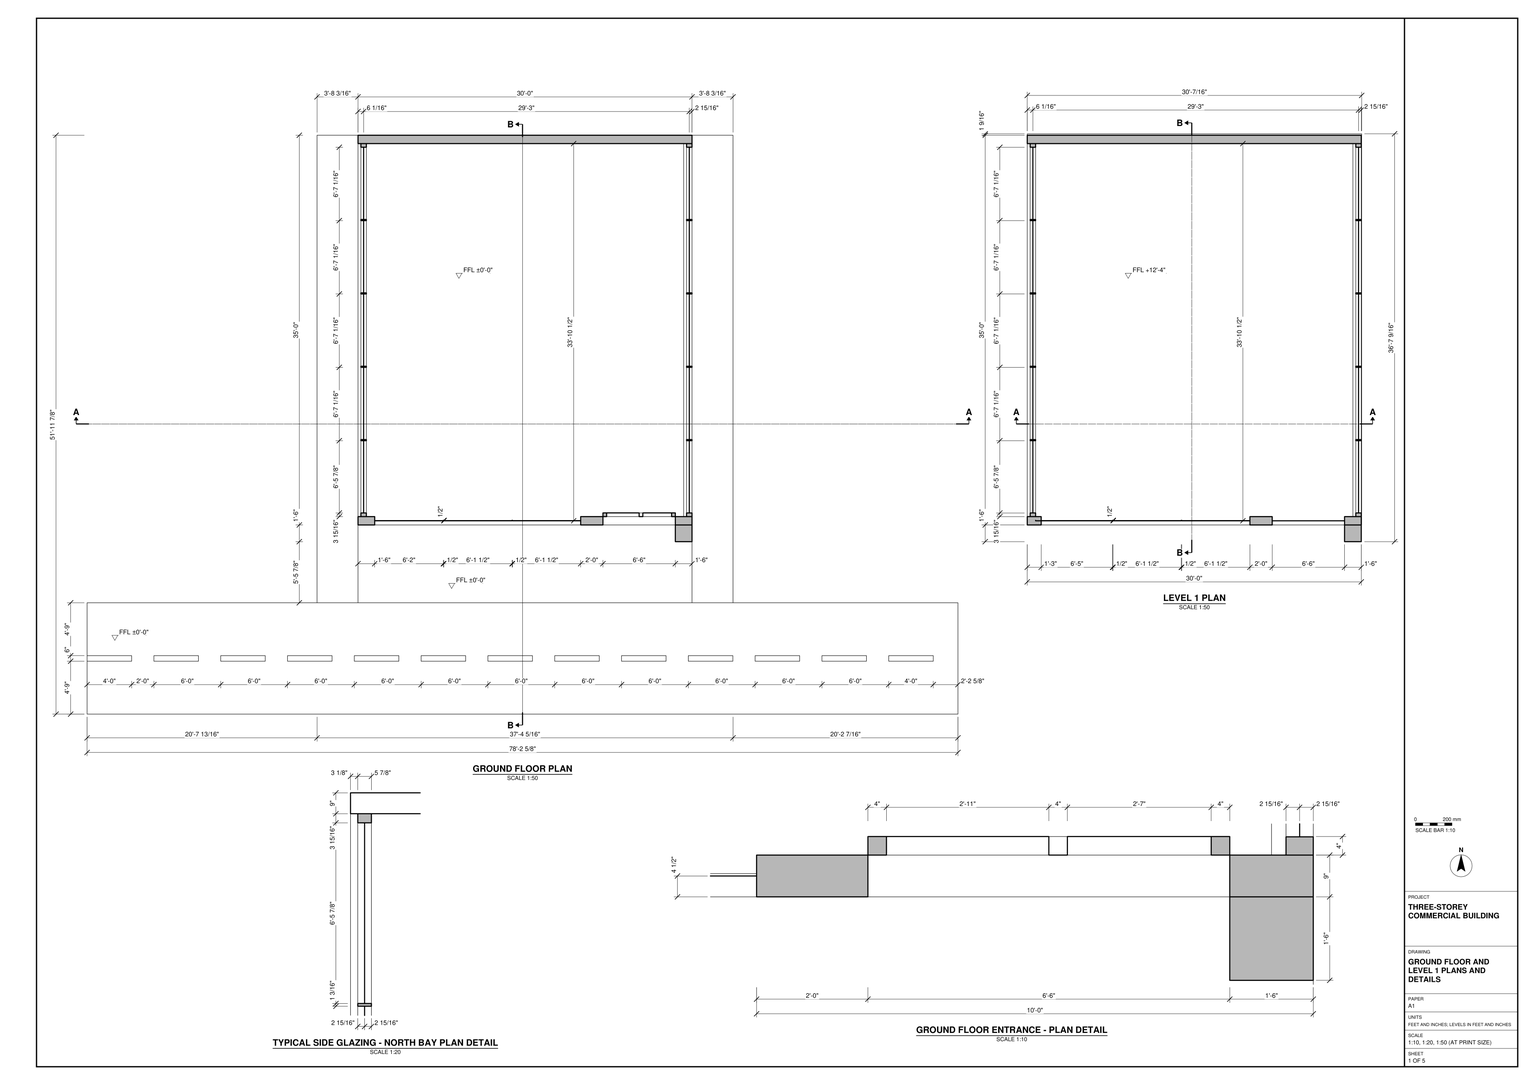
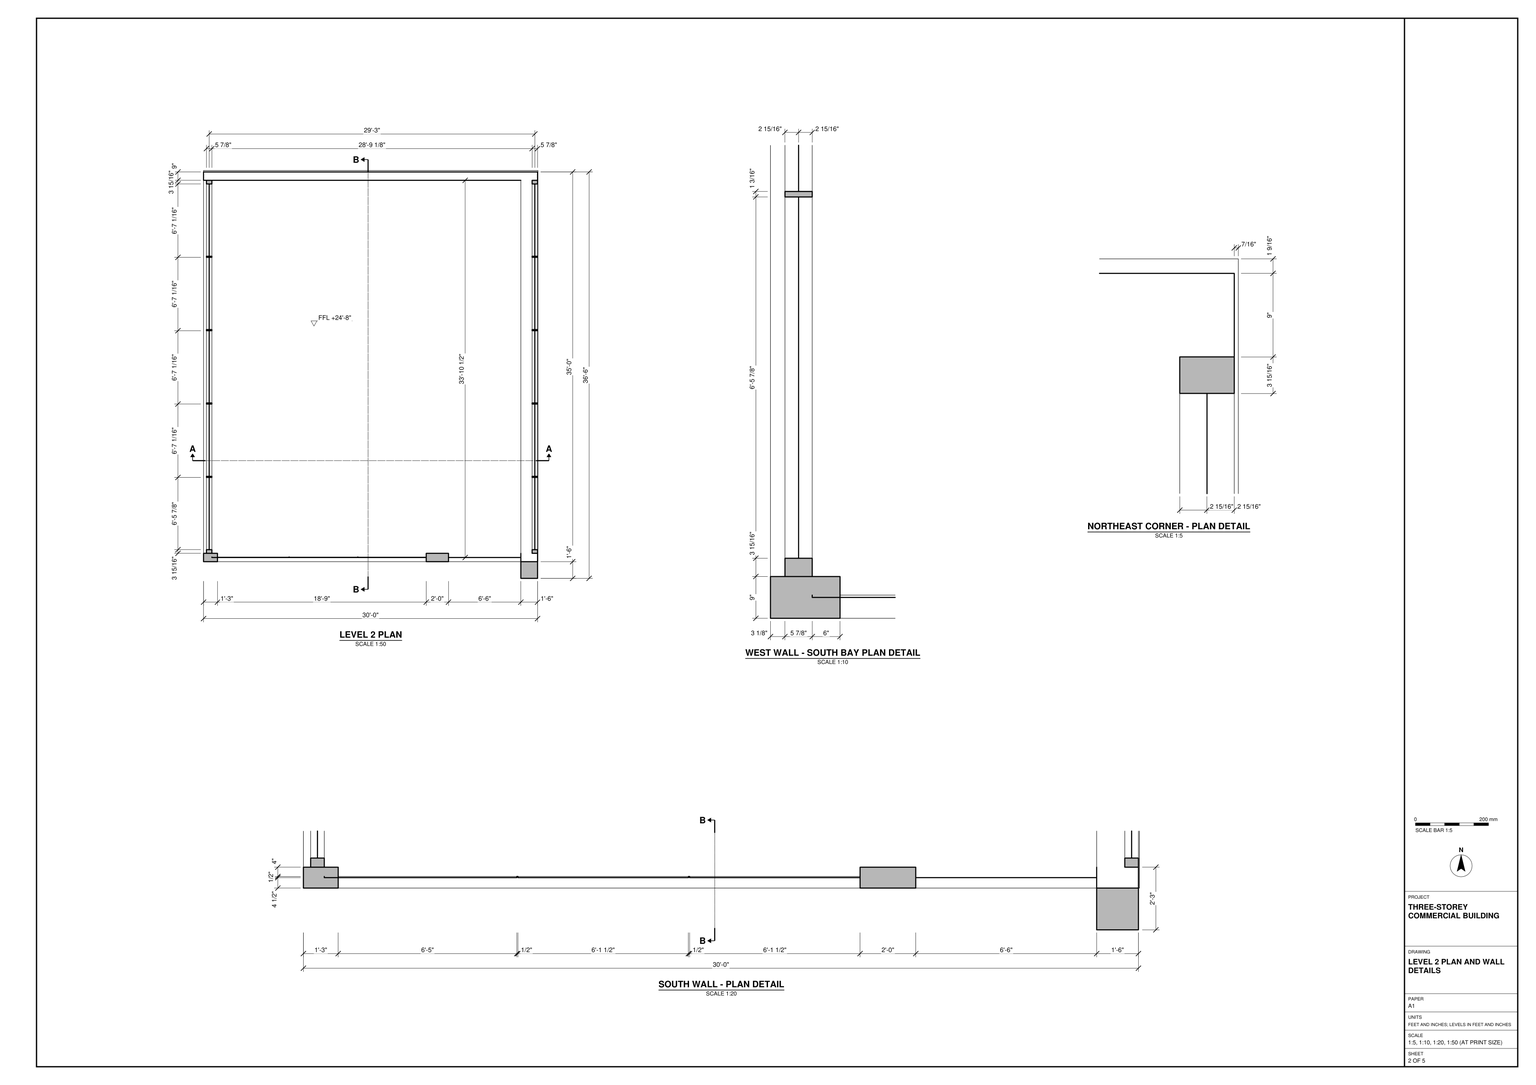
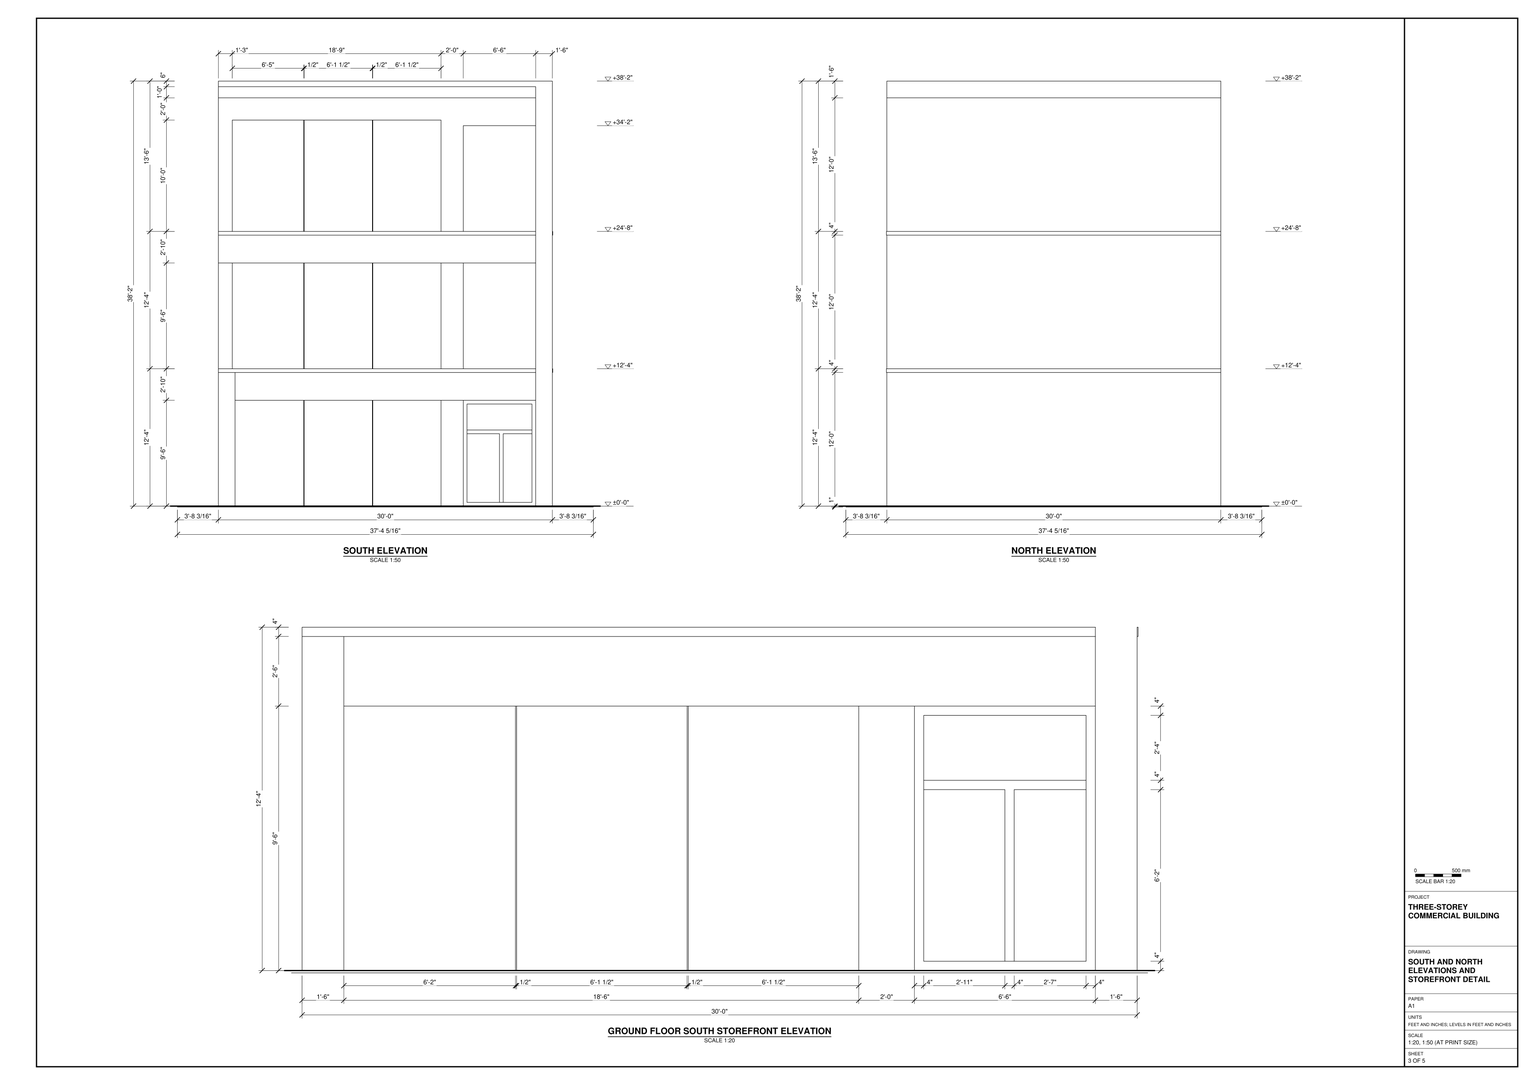
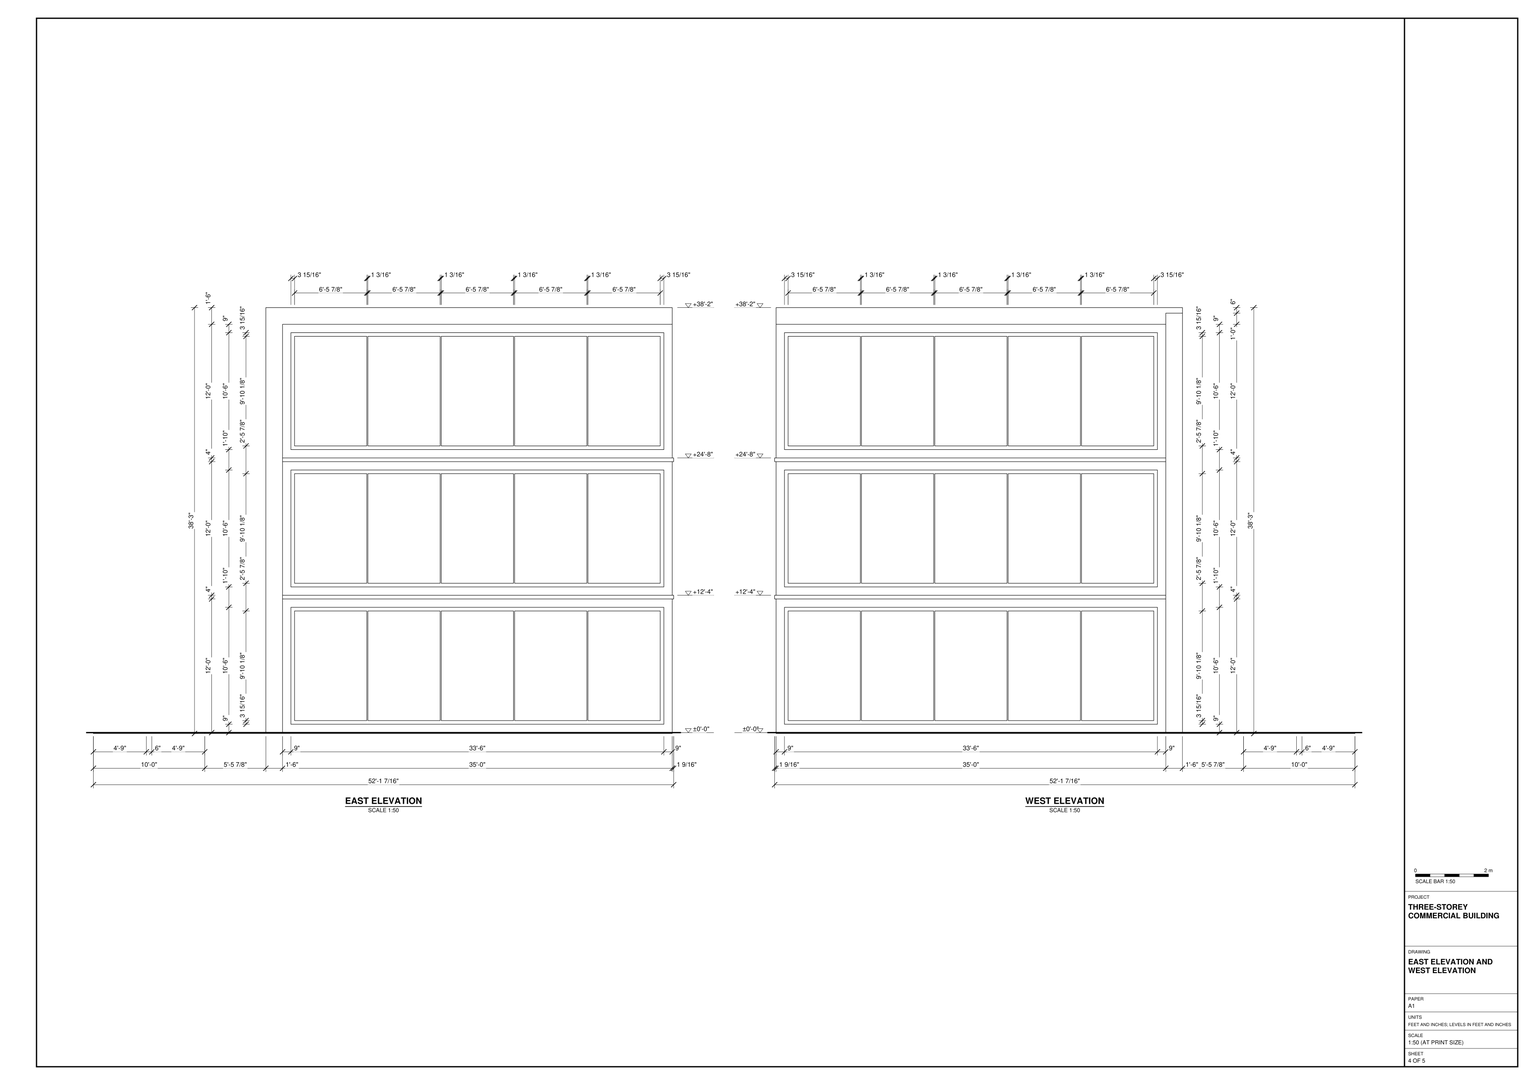
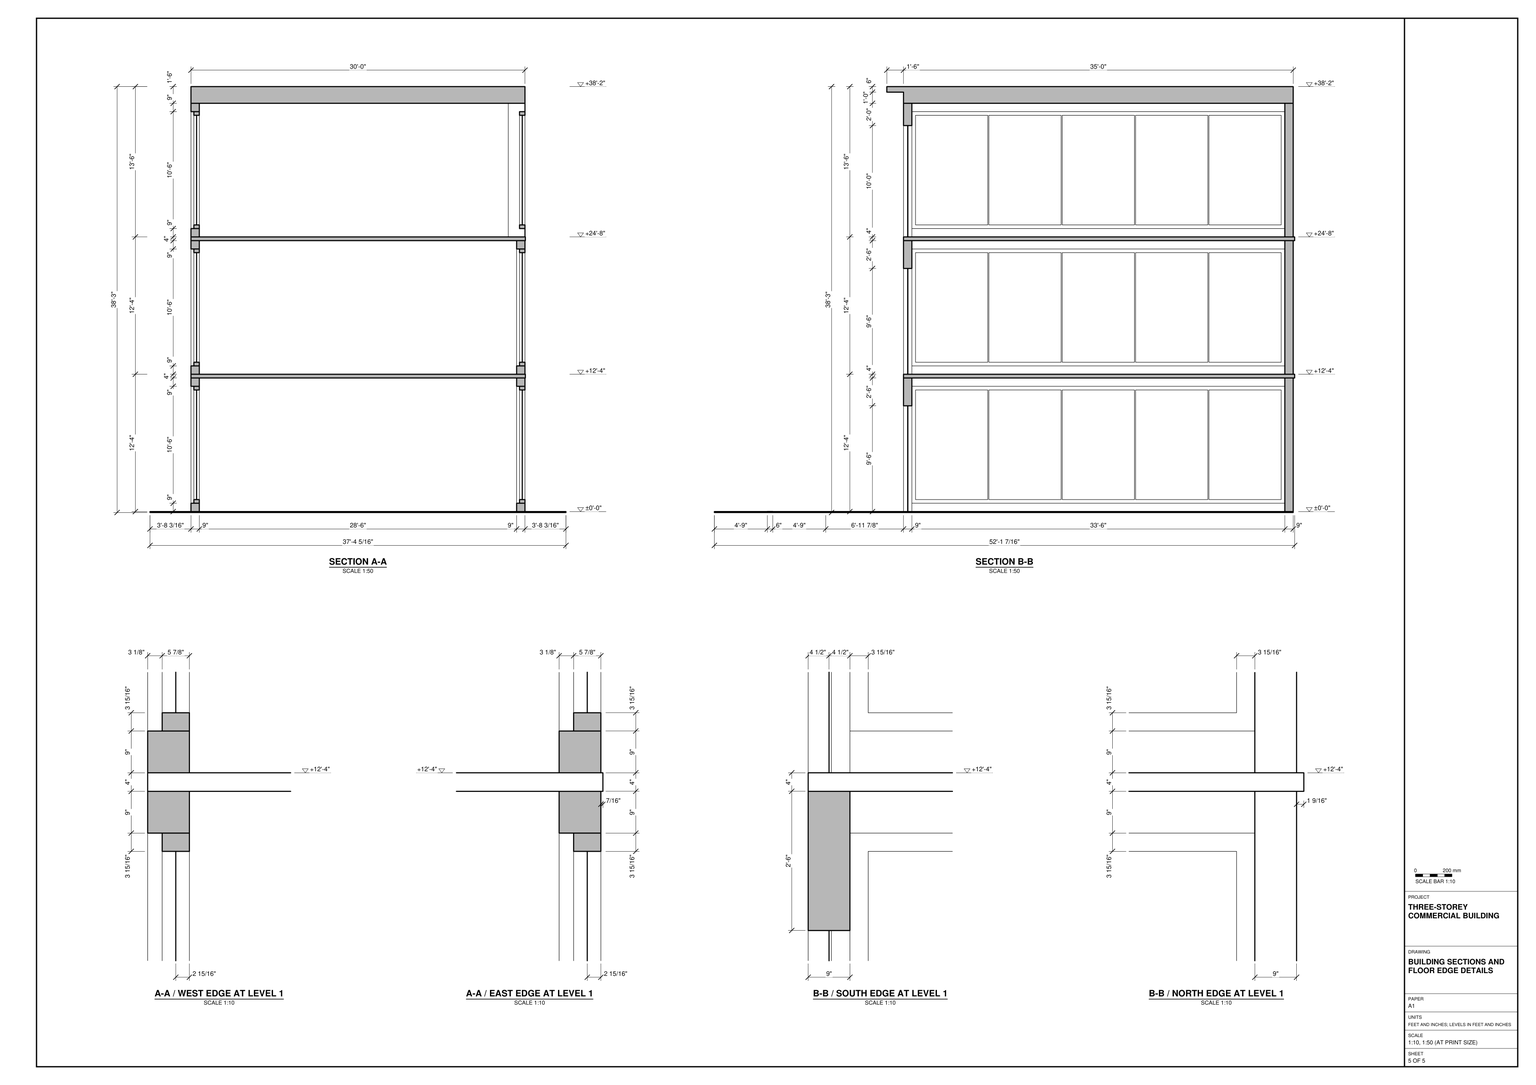
Build the commercial building and its street frontage in SketchUp using task_files/diagram_01.pdf. Work in feet and inches. Including the site base and road, the overall model extents are 78'-2 5/8" along X, 52'-1 7/16" along Y and 38'-3" along Z. Set the finished floor levels at ±0'-0", +12'-4" and +24'-8".

Set the rectangular building back from the road with the storefront facing south. Extend the road beyond both sides of the site base and include its dashed centre markings. Model the open floor plates, floor slabs, perimeter walls and flat roof. Follow the plan details for wall thicknesses, glazing positions, mullions and corner returns. Keep the north wall solid and carry the repeated glazing bays along the east and west sides. On the ground-floor south elevation, place the broad display glazing to the left of the entrance and include the entrance frame and transom. Follow the upper elevations for the window divisions and solid bands between storeys.

Keep walls, slabs, roof and site elements in separate groups or components. Keep each furniture or joinery piece shown separate and use components for repeated parts. Any decor or loose items shown may be represented by suitable library components. Save one SketchUp model as output_files/three_storey_commercial_building_with_glazed_storefront.skp.

# SketchUp Ruby script. Lengths in inches.
U = 1.inch
M = Sketchup.active_model
def pt(a) = Geom::Point3d.new(a.map { |v| v * U })
def face(e, loops, mat)
  f = e.add_face(loops[0].map { |a| pt(a) })
  loops[1..].each { |l| e.add_face(l.map { |a| pt(a) }).erase! }
  f.material = f.back_material = mat if mat
  f
end
# faces: each face lists its corners as indices into pts; further lists are holes
def faces(e, pts, list, mat = nil) = list.each { |f| face(e, (f[0].is_a?(Array) ? f : [f]).map { |l| l.map { |i| pts[i] } }, mat) }
# xy, xz, yz: faces in a plane at the given z, y or x. An outline is a flat list of corners, or four numbers for a rectangle; further outlines are holes
def ring(l) = l.size == 4 ? [[l[0], l[1]], [l[2], l[1]], [l[2], l[3]], [l[0], l[3]]] : l.each_slice(2).to_a
def flat(e, list, mat, &to3) = list.each { |f| face(e, (f[0].is_a?(Array) ? f : [f]).map { |l| ring(l).map { |u, v| to3.(u, v) } }, mat) }
def xy(e, z, list, mat = nil) = flat(e, list, mat) { |x, y| [x, y, z] }
def xz(e, y, list, mat = nil) = flat(e, list, mat) { |x, z| [x, y, z] }
def yz(e, x, list, mat = nil) = flat(e, list, mat) { |y, z| [x, y, z] }
def lines(e, pts, list) = list.each { |a, b| e.add_line(pt(pts[a]), pt(pts[b])) }
# prism: a flat outline (further loops are holes) pulled along v
def prism(e, loops, v, mat = nil)
  f = face(e, loops, mat); d = Geom::Vector3d.new(v.map { |x| x * U })
  f.pushpull(f.normal.samedirection?(d) ? d.length : -d.length)
end
def box(e, o, s, mat = nil) = prism(e, [[o, [o[0] + s[0], o[1], o[2]], [o[0] + s[0], o[1] + s[1], o[2]], [o[0], o[1] + s[1], o[2]]]], [0, 0, s[2]], mat)
def at(x, y, z, deg = 0) = Geom::Transformation.translation(pt([x, y, z])) * Geom::Transformation.rotation(ORIGIN, Z_AXIS, deg.degrees)
def axes(o, x, y, z) = Geom::Transformation.new([*x, 0, *y, 0, *z, 0, *pt(o).to_a, 1])
def part(name) = M.definitions.add(name)
# library, detail: a bought-in or finely detailed component or shape, given as its bounding box
def library(name, o, s) = part(name).tap { |d| box(d.entities, o, s) }
def detail(e, o, s) = box(e.add_group.entities, o, s)
def put(e, d, t, mat = nil) = e.add_instance(d, t).tap { |i| i.material = mat if mat }
def group(e, t, mat = nil) = e.add_group.tap { |g| g.transformation = t; g.material = mat if mat }.entities
root = M.entities
M.materials.add("[Color E01]").color = [255, 255, 204]
M.materials.add("[Color L04]").color = [255, 50, 152]
M.materials.add("[Color M06]").color = [86, 86, 86]
M.materials.add("[Color M08]").color = [30, 30, 30]
M.materials.add("[Marble Carrara Gold Floor Tile]").color = [225, 223, 217]
M.materials.add("[Translucent Glass Gray]").color = [128, 128, 128]
M.materials["[Translucent Glass Gray]"].alpha = 0.5
c1 = part("Group\#4")
xy(c1.entities,0,[[0,0,360.4375,421.5625]])
xy(c1.entities,4,[[0,0,360.4375,421.5625]])
xz(c1.entities,0,[[0,0,360.4375,4]],"[Color M06]")
xz(c1.entities,421.5625,[[0,0,360.4375,4]])
yz(c1.entities,0,[[0,0,421.5625,4]])
yz(c1.entities,360.4375,[[0,0,421.5625,4]])
c2 = part("Group\#3")
xy(c2.entities,0,[[-9,0,74,0.5],[74.5,0,148,0.5],[148.5,0,222,0.5]],"[Translucent Glass Gray]")
xy(c2.entities,114,[[-9,0,74,0.5],[74.5,0,148,0.5],[148.5,0,222,0.5]],"[Translucent Glass Gray]")
xz(c2.entities,0,[[-9,0,74,114],[74.5,0,148,114],[148.5,0,222,114]],"[Translucent Glass Gray]")
xz(c2.entities,0.5,[[74,0,74.5,114],[148,0,148.5,114]],"[Translucent Glass Gray]")
yz(c2.entities,-9,[[0,0,0.5,114]],"[Translucent Glass Gray]")
yz(c2.entities,74,[[0,0,0.5,114]],"[Translucent Glass Gray]")
yz(c2.entities,74.5,[[0,0,0.5,114]],"[Translucent Glass Gray]")
yz(c2.entities,148,[[0,0,0.5,114]],"[Translucent Glass Gray]")
yz(c2.entities,148.5,[[0,0,0.5,114]],"[Translucent Glass Gray]")
yz(c2.entities,222,[[0,0,0.5,114]],"[Translucent Glass Gray]")
c3 = part("Group\#11")
xz(c3.entities,0,[[0,0,78,114]])
c4 = part("Group\#13")
box(c4.entities,[0,0,0],[48,6,0.1])
c5 = part("Group17\#2")
xy(c5.entities,0,[[-197.0625,-59.0625,-119.1875,59.0625],[-118,-59.0625,-40.125,59.0625],[-38.9375,-59.0625,38.9375,59.0625],[40.125,-59.0625,118,59.0625],[119.1875,-59.0625,197.0625,59.0625]])
c6 = part("Group16\#1")
xy(c6.entities,0,[[[-201,-63,201,63],[-118,-59.0625,-40.125,59.0625],[40.125,-59.0625,118,59.0625],[-38.9375,-59.0625,38.9375,59.0625],[119.1875,-59.0625,197.0625,59.0625],[-197.0625,-59.0625,-119.1875,59.0625]]])
xy(c6.entities,5.875,[[[-201,-63,201,63],[40.125,-59.0625,118,59.0625],[-118,-59.0625,-40.125,59.0625],[-38.9375,-59.0625,38.9375,59.0625],[119.1875,-59.0625,197.0625,59.0625],[-197.0625,-59.0625,-119.1875,59.0625]]],"[Color M08]")
xz(c6.entities,-63,[[-201,0,201,5.875]])
xz(c6.entities,-59.0625,[[-197.0625,0,-119.1875,5.875],[-118,0,-40.125,5.875],[-38.9375,0,38.9375,5.875],[40.125,0,118,5.875],[119.1875,0,197.0625,5.875]])
xz(c6.entities,59.0625,[[-197.0625,0,-119.1875,5.875],[-118,0,-40.125,5.875],[-38.9375,0,38.9375,5.875],[40.125,0,118,5.875],[119.1875,0,197.0625,5.875]])
xz(c6.entities,63,[[-201,0,201,5.875]])
yz(c6.entities,-201,[[-63,0,63,5.875]])
yz(c6.entities,-197.0625,[[-59.0625,0,59.0625,5.875]])
yz(c6.entities,-119.1875,[[-59.0625,0,59.0625,5.875]])
yz(c6.entities,-118,[[-59.0625,0,59.0625,5.875]])
yz(c6.entities,-40.125,[[-59.0625,0,59.0625,5.875]])
yz(c6.entities,-38.9375,[[-59.0625,0,59.0625,5.875]])
yz(c6.entities,38.9375,[[-59.0625,0,59.0625,5.875]])
yz(c6.entities,40.125,[[-59.0625,0,59.0625,5.875]])
yz(c6.entities,118,[[-59.0625,0,59.0625,5.875]])
yz(c6.entities,119.1875,[[-59.0625,0,59.0625,5.875]])
yz(c6.entities,197.0625,[[-59.0625,0,59.0625,5.875]])
yz(c6.entities,201,[[-63,0,63,5.875]])
put(c6.entities,c5,at(0,0,2.9375),"[Translucent Glass Gray]")
c7 = part("Group19\#2")
xy(c7.entities,0,[[-197.0625,-59.0625,-119.1875,59.0625],[-118,-59.0625,-40.125,59.0625],[-38.9375,-59.0625,38.9375,59.0625],[40.125,-59.0625,118,59.0625],[119.1875,-59.0625,197.0625,59.0625]])
c8 = part("Group18\#2")
xy(c8.entities,0,[[[-201,-63,201,63],[-197.0625,-59.0625,-119.1875,59.0625],[-118,-59.0625,-40.125,59.0625],[-38.9375,-59.0625,38.9375,59.0625],[40.125,-59.0625,118,59.0625],[119.1875,-59.0625,197.0625,59.0625]]])
xy(c8.entities,5.875,[[[-201,-63,201,63],[40.125,-59.0625,118,59.0625],[-197.0625,-59.0625,-119.1875,59.0625],[-118,-59.0625,-40.125,59.0625],[-38.9375,-59.0625,38.9375,59.0625],[119.1875,-59.0625,197.0625,59.0625]]],"[Color M08]")
xz(c8.entities,-63,[[-201,0,201,5.875]])
xz(c8.entities,-59.0625,[[-197.0625,0,-119.1875,5.875],[-118,0,-40.125,5.875],[-38.9375,0,38.9375,5.875],[40.125,0,118,5.875],[119.1875,0,197.0625,5.875]])
xz(c8.entities,59.0625,[[-197.0625,0,-119.1875,5.875],[-118,0,-40.125,5.875],[-38.9375,0,38.9375,5.875],[40.125,0,118,5.875],[119.1875,0,197.0625,5.875]])
xz(c8.entities,63,[[-201,0,201,5.875]])
yz(c8.entities,-201,[[-63,0,63,5.875]])
yz(c8.entities,-197.0625,[[-59.0625,0,59.0625,5.875]])
yz(c8.entities,-119.1875,[[-59.0625,0,59.0625,5.875]])
yz(c8.entities,-118,[[-59.0625,0,59.0625,5.875]])
yz(c8.entities,-40.125,[[-59.0625,0,59.0625,5.875]])
yz(c8.entities,-38.9375,[[-59.0625,0,59.0625,5.875]])
yz(c8.entities,38.9375,[[-59.0625,0,59.0625,5.875]])
yz(c8.entities,40.125,[[-59.0625,0,59.0625,5.875]])
yz(c8.entities,118,[[-59.0625,0,59.0625,5.875]])
yz(c8.entities,119.1875,[[-59.0625,0,59.0625,5.875]])
yz(c8.entities,197.0625,[[-59.0625,0,59.0625,5.875]])
yz(c8.entities,201,[[-63,0,63,5.875]])
put(c8.entities,c7,at(0,0,2.9375),"[Translucent Glass Gray]")
c9 = part("Group18\#1")
xy(c9.entities,0,[[[-201,-63,201,63],[-197.0625,-59.0625,-119.1875,59.0625],[-118,-59.0625,-40.125,59.0625],[40.125,-59.0625,118,59.0625],[-38.9375,-59.0625,38.9375,59.0625],[119.1875,-59.0625,197.0625,59.0625]]],"[Color M08]")
xy(c9.entities,5.875,[[[-201,-63,201,63],[-197.0625,-59.0625,-119.1875,59.0625],[40.125,-59.0625,118,59.0625],[-118,-59.0625,-40.125,59.0625],[-38.9375,-59.0625,38.9375,59.0625],[119.1875,-59.0625,197.0625,59.0625]]],"[Color M08]")
xz(c9.entities,-63,[[-201,0,201,5.875]])
xz(c9.entities,-59.0625,[[-197.0625,0,-119.1875,5.875],[-118,0,-40.125,5.875],[-38.9375,0,38.9375,5.875],[40.125,0,118,5.875],[119.1875,0,197.0625,5.875]])
xz(c9.entities,59.0625,[[-197.0625,0,-119.1875,5.875],[-118,0,-40.125,5.875],[-38.9375,0,38.9375,5.875],[40.125,0,118,5.875],[119.1875,0,197.0625,5.875]])
xz(c9.entities,63,[[-201,0,201,5.875]])
yz(c9.entities,-201,[[-63,0,63,5.875]])
yz(c9.entities,-197.0625,[[-59.0625,0,59.0625,5.875]])
yz(c9.entities,-119.1875,[[-59.0625,0,59.0625,5.875]])
yz(c9.entities,-118,[[-59.0625,0,59.0625,5.875]])
yz(c9.entities,-40.125,[[-59.0625,0,59.0625,5.875]])
yz(c9.entities,-38.9375,[[-59.0625,0,59.0625,5.875]])
yz(c9.entities,38.9375,[[-59.0625,0,59.0625,5.875]])
yz(c9.entities,40.125,[[-59.0625,0,59.0625,5.875]])
yz(c9.entities,118,[[-59.0625,0,59.0625,5.875]])
yz(c9.entities,119.1875,[[-59.0625,0,59.0625,5.875]])
yz(c9.entities,197.0625,[[-59.0625,0,59.0625,5.875]])
yz(c9.entities,201,[[-63,0,63,5.875]])
put(c9.entities,c7,at(0,0,2.9375),"[Translucent Glass Gray]")
p = [[651.98,614.86,283],[651.98,212.86,283],[651.98,212.86,157],[651.98,614.86,157]]
lines(root,p,[[0,1],[1,2],[2,3],[3,0]])
g1 = group(root,at(291.98,203.86,0))
xy(g1,0,[[0,0,0,420,360,420,360,0,342,0,342,9,351,9,351,411,9,411,9,9,18,9,18,0],[240,0,264,9]])
xy(g1,9,[[0,9,9,411],[351,9,360,411]])
xy(g1,114,[[18,0,240,9],[264,0,342,9]])
xy(g1,135,[[0,9,9,411],[351,9,360,411]])
xy(g1,144,[[[0,0,360,420],[9,9,351,411]]])
xz(g1,0,[[0,0,18,144],[240,0,264,114],[342,0,360,144],[18,114,342,144]],"[Color M06]")
xz(g1,9,[[9,0,9,144,351,144,351,0,342,0,342,114,264,114,264,0,240,0,240,114,18,114,18,0],[0,9,9,135],[351,9,360,135]])
xz(g1,411,[[9,0,351,144],[0,9,9,135],[351,9,360,135]])
xz(g1,420,[[0,0,360,144]])
yz(g1,0,[[[0,0,420,144],[9,9,411,135]]])
yz(g1,9,[[9,0,411,9],[9,135,411,144]])
yz(g1,18,[[0,0,9,114]])
yz(g1,240,[[0,0,9,114]])
yz(g1,264,[[0,0,9,114]])
yz(g1,342,[[0,0,9,114]])
yz(g1,351,[[9,0,411,9],[9,135,411,144]])
yz(g1,360,[[[0,0,420,144],[9,9,411,135]]])
g2 = group(g1,at(264,9,0))
xy(g2,0,[[0,0,78,4]])
xy(g2,4,[[4,0,39,4],[39,0,43,4],[43,0,74,4]])
xy(g2,78,[[4,0,39,4],[43,0,74,4]])
xy(g2,82,[[4,0,74,4]])
xy(g2,110,[[4,0,74,4]])
xy(g2,114,[[0,0,78,4]])
xz(g2,0,[[[0,0,78,114],[4,4,74,110]],[39,4,43,4,43,78,74,78,74,82,4,82,4,78,39,78]],"[Color M08]")
xz(g2,4,[[[0,0,78,114],[4,4,74,110]]])
xz(g2,4,[[4,4,39,78],[43,4,74,78],[4,82,74,110]],"[Translucent Glass Gray]")
yz(g2,0,[[0,0,4,114]])
yz(g2,4,[[0,4,4,78],[0,78,4,82],[0,82,4,110]])
yz(g2,39,[[0,4,4,78]])
yz(g2,43,[[0,4,4,78]])
yz(g2,74,[[0,4,4,78],[0,78,4,82],[0,82,4,110]])
yz(g2,78,[[0,0,4,114]])
g3 = group(g1,at(18,4.5,0))
xy(g3,0,[[0,0,74,0.5],[74.5,0,148,0.5],[148.5,0,222,0.5]],"[Translucent Glass Gray]")
xy(g3,114,[[0,0,74,0.5],[74.5,0,148,0.5],[148.5,0,222,0.5]],"[Translucent Glass Gray]")
xz(g3,0,[[0,0,74,114],[74.5,0,148,114],[148.5,0,222,114]],"[Translucent Glass Gray]")
xz(g3,0.5,[[74,0,74.5,114],[148,0,148.5,114]],"[Translucent Glass Gray]")
yz(g3,0,[[0,0,0.5,114]],"[Translucent Glass Gray]")
yz(g3,74,[[0,0,0.5,114]],"[Translucent Glass Gray]")
yz(g3,74.5,[[0,0,0.5,114]],"[Translucent Glass Gray]")
yz(g3,148,[[0,0,0.5,114]],"[Translucent Glass Gray]")
yz(g3,148.5,[[0,0,0.5,114]],"[Translucent Glass Gray]")
yz(g3,222,[[0,0,0.5,114]],"[Translucent Glass Gray]")
put(root,c1,at(291.98,203.86,144))
g4 = group(root,at(291.98,203.86,-1))
box(g4,[0,0,0],[360,420,1])
g5 = group(root,at(291.98,159.6875,-1),"[Marble Carrara Gold Floor Tile]")
box(g5,[0,-39.6875,0],[360,83.86,1])
g6 = group(root,at(651.98,519.6875,-1,-90),"[Marble Carrara Gold Floor Tile]")
box(g6,[-104.17,0,0],[503.86,44.17,1])
g7 = group(root,at(247.8125,519.6875,-1,-90),"[Marble Carrara Gold Floor Tile]")
box(g7,[-104.17,0,0],[503.86,44.17,1])
g8 = group(root,at(291.98,203.86,148))
xy(g8,0,[[0,0,0,420,360,420,360,0,342,0,342,9,351,9,351,411,9,411,9,9,15,9,15,0],[240,0,264,9]])
xy(g8,9,[[0,9,9,411],[351,9,360,411]])
xy(g8,114,[[15,0,240,9],[264,0,342,9]])
xy(g8,135,[[0,9,9,411],[351,9,360,411]])
xy(g8,144,[[[0,0,360,420],[9,9,351,411]]])
xz(g8,0,[[0,0,15,114],[240,0,264,114]],"[Color E01]")
xz(g8,0,[[342,0,360,144],[0,114,342,144]],"[Color M06]")
xz(g8,9,[[240,0,240,114,9,114,9,144,351,144,351,0,342,0,342,114,264,114,264,0],[9,0,15,114],[0,9,9,114],[351,9,360,135],[0,114,9,135]])
xz(g8,411,[[9,0,351,144],[0,9,9,135],[351,9,360,135]])
xz(g8,420,[[0,0,360,144]])
yz(g8,0,[[[0,0,420,144],[9,9,411,135]]])
yz(g8,9,[[9,0,411,9],[9,135,411,144]])
yz(g8,15,[[0,0,9,114]])
yz(g8,240,[[0,0,9,114]])
yz(g8,264,[[0,0,9,114]])
yz(g8,342,[[0,0,9,114]])
yz(g8,351,[[9,0,411,9],[9,135,411,144]])
yz(g8,360,[[[0,0,420,144],[9,9,411,135]]])
put(g8,c2,at(18,4.5,0))
put(root,c3,at(555.98,208.36,148),"[Translucent Glass Gray]")
g9 = group(root,at(0,0,-1),"[Color M08]")
box(g9,[0,0,0],[938.61,120,1])
put(root,c4,at(0,57,0))
put(root,c4,at(72,57,0))
put(root,c4,at(144,57,0))
put(root,c4,at(216,57,0))
put(root,c4,at(288,57,0))
put(root,c4,at(360,57,0))
put(root,c4,at(432,57,0))
put(root,c4,at(504,57,0))
put(root,c4,at(576,57,0))
put(root,c4,at(648,57,0))
put(root,c4,at(720,57,0))
put(root,c4,at(792,57,0))
put(root,c4,at(864,57,0))
g10 = group(root,at(291.98,203.86,296))
xy(g10,0,[[0,0,0,420,360,420,360,0,342,0,342,411,9,411,9,9,15,9,15,0],[240,0,264,9]])
xy(g10,9,[[0,9,9,411]])
xy(g10,114,[[264,0,342,9]])
xy(g10,120,[[15,0,240,9]])
xy(g10,135,[[0,9,9,411]])
xy(g10,144,[[[0,0,360,420],[9,9,342,411]]])
xz(g10,0,[[0,0,15,0,15,120,240,120,240,0,264,0,264,114,342,114,342,144,0,144]],"[Color E01]")
xz(g10,0,[[342,0,360,144]],"[Color M06]")
xz(g10,9,[[240,0,240,120,15,120,15,114,9,114,9,144,342,144,342,114,264,114,264,0],[9,0,15,114],[0,9,9,135]])
xz(g10,411,[[9,0,342,144],[0,9,9,135]])
xz(g10,420,[[0,0,360,144]])
yz(g10,0,[[[0,0,420,144],[9,9,411,135]]])
yz(g10,9,[[9,0,411,9],[9,135,411,144]])
yz(g10,15,[[0,0,9,120]])
yz(g10,240,[[0,0,9,120]])
yz(g10,264,[[0,0,9,114]])
yz(g10,342,[[0,0,9,114]])
yz(g10,360,[[[0,0,420,144],[9,9,411,135]]])
put(g10,c2,axes([18,4.5,0],[1,0,0],[0,1,0],[0,0,1.05263]))
put(g10,c6,axes([354.125,210,72],[0,1,0],[0,0,1],[1,0,0]))
put(root,c1,at(291.98,203.86,292))
g11 = group(root,at(291.98,185.86,0),"[Color M06]")
xy(g11,0,[[342,0,360,18]])
xy(g11,440,[[[0,18,360,438],[119.6,351.17,122.72,351.39,125.68,352.41,128.28,354.17,130.33,356.54,131.7,359.35,132.29,362.43,132.07,365.55,131.05,368.51,129.29,371.11,126.93,373.16,124.11,374.53,121.03,375.125,117.91,374.9,114.95,373.88,112.35,372.125,110.3,369.76,108.93,366.94,108.34,363.87,108.56,360.74,109.58,357.78,111.34,355.18,113.7,353.13,116.52,351.76],[119.6,303.17,122.72,303.39,125.68,304.41,128.28,306.17,130.33,308.54,131.7,311.35,132.29,314.43,132.07,317.55,131.05,320.51,129.29,323.11,126.93,325.16,124.11,326.53,121.03,327.125,117.91,326.9,114.95,325.88,112.35,324.125,110.3,321.76,108.93,318.94,108.34,315.87,108.56,312.74,109.58,309.78,111.34,307.18,113.7,305.13,116.52,303.76],[119.6,255.17,122.72,255.39,125.68,256.41,128.28,258.17,130.33,260.54,131.7,263.35,132.29,266.43,132.07,269.55,131.05,272.51,129.29,275.11,126.93,277.16,124.11,278.53,121.03,279.125,117.91,278.9,114.95,277.88,112.35,276.125,110.3,273.76,108.93,270.94,108.34,267.87,108.56,264.74,109.58,261.78,111.34,259.18,113.7,257.13,116.52,255.76],[119.6,207.17,122.72,207.39,125.68,208.41,128.28,210.17,130.33,212.54,131.7,215.35,132.29,218.43,132.07,221.55,131.05,224.51,129.29,227.11,126.93,229.16,124.11,230.53,121.03,231.125,117.91,230.9,114.95,229.88,112.35,228.125,110.3,225.76,108.93,222.94,108.34,219.87,108.56,216.74,109.58,213.78,111.34,211.18,113.7,209.13,116.52,207.76],[119.6,159.17,122.72,159.39,125.68,160.41,128.28,162.17,130.33,164.54,131.7,167.35,132.29,170.43,132.07,173.55,131.05,176.51,129.29,179.11,126.93,181.16,124.11,182.53,121.03,183.125,117.91,182.9,114.95,181.88,112.35,180.125,110.3,177.76,108.93,174.94,108.34,171.87,108.56,168.74,109.58,165.78,111.34,163.18,113.7,161.13,116.52,159.76],[119.6,111.17,122.72,111.39,125.68,112.41,128.28,114.17,130.33,116.54,131.7,119.35,132.29,122.43,132.07,125.55,131.05,128.51,129.29,131.11,126.93,133.16,124.11,134.53,121.03,135.125,117.91,134.9,114.95,133.88,112.35,132.125,110.3,129.76,108.93,126.94,108.34,123.87,108.56,120.74,109.58,117.78,111.34,115.18,113.7,113.13,116.52,111.76],[119.6,63.17,122.72,63.39,125.68,64.41,128.28,66.17,130.33,68.54,131.7,71.35,132.29,74.43,132.07,77.55,131.05,80.51,129.29,83.11,126.93,85.16,124.11,86.53,121.03,87.125,117.91,86.9,114.95,85.88,112.35,84.125,110.3,81.76,108.93,78.94,108.34,75.87,108.56,72.74,109.58,69.78,111.34,67.18,113.7,65.13,116.52,63.76],[47.6,303.17,50.72,303.39,53.68,304.41,56.28,306.17,58.33,308.54,59.7,311.35,60.29,314.43,60.07,317.55,59.05,320.51,57.29,323.11,54.93,325.16,52.11,326.53,49.03,327.125,45.91,326.9,42.95,325.88,40.35,324.125,38.3,321.76,36.93,318.94,36.34,315.87,36.56,312.74,37.58,309.78,39.34,307.18,41.7,305.13,44.52,303.76],[47.6,255.17,50.72,255.39,53.68,256.41,56.28,258.17,58.33,260.54,59.7,263.35,60.29,266.43,60.07,269.55,59.05,272.51,57.29,275.11,54.93,277.16,52.11,278.53,49.03,279.125,45.91,278.9,42.95,277.88,40.35,276.125,38.3,273.76,36.93,270.94,36.34,267.87,36.56,264.74,37.58,261.78,39.34,259.18,41.7,257.13,44.52,255.76],[47.6,207.17,50.72,207.39,53.68,208.41,56.28,210.17,58.33,212.54,59.7,215.35,60.29,218.43,60.07,221.55,59.05,224.51,57.29,227.11,54.93,229.16,52.11,230.53,49.03,231.125,45.91,230.9,42.95,229.88,40.35,228.125,38.3,225.76,36.93,222.94,36.34,219.87,36.56,216.74,37.58,213.78,39.34,211.18,41.7,209.13,44.52,207.76],[47.6,159.17,50.72,159.39,53.68,160.41,56.28,162.17,58.33,164.54,59.7,167.35,60.29,170.43,60.07,173.55,59.05,176.51,57.29,179.11,54.93,181.16,52.11,182.53,49.03,183.125,45.91,182.9,42.95,181.88,40.35,180.125,38.3,177.76,36.93,174.94,36.34,171.87,36.56,168.74,37.58,165.78,39.34,163.18,41.7,161.13,44.52,159.76],[47.6,111.17,50.72,111.39,53.68,112.41,56.28,114.17,58.33,116.54,59.7,119.35,60.29,122.43,60.07,125.55,59.05,128.51,57.29,131.11,54.93,133.16,52.11,134.53,49.03,135.125,45.91,134.9,42.95,133.88,40.35,132.125,38.3,129.76,36.93,126.94,36.34,123.87,36.56,120.74,37.58,117.78,39.34,115.18,41.7,113.13,44.52,111.76],[47.6,63.17,50.72,63.39,53.68,64.41,56.28,66.17,58.33,68.54,59.7,71.35,60.29,74.43,60.07,77.55,59.05,80.51,57.29,83.11,54.93,85.16,52.11,86.53,49.03,87.125,45.91,86.9,42.95,85.88,40.35,84.125,38.3,81.76,36.93,78.94,36.34,75.87,36.56,72.74,37.58,69.78,39.34,67.18,41.7,65.13,44.52,63.76],[191.6,351.17,194.72,351.39,197.68,352.41,200.28,354.17,202.33,356.54,203.7,359.35,204.29,362.43,204.07,365.55,203.05,368.51,201.29,371.11,198.93,373.16,196.11,374.53,193.03,375.125,189.91,374.9,186.95,373.88,184.35,372.125,182.3,369.76,180.93,366.94,180.34,363.87,180.56,360.74,181.58,357.78,183.34,355.18,185.7,353.13,188.52,351.76],[191.6,303.17,194.72,303.39,197.68,304.41,200.28,306.17,202.33,308.54,203.7,311.35,204.29,314.43,204.07,317.55,203.05,320.51,201.29,323.11,198.93,325.16,196.11,326.53,193.03,327.125,189.91,326.9,186.95,325.88,184.35,324.125,182.3,321.76,180.93,318.94,180.34,315.87,180.56,312.74,181.58,309.78,183.34,307.18,185.7,305.13,188.52,303.76],[191.6,255.17,194.72,255.39,197.68,256.41,200.28,258.17,202.33,260.54,203.7,263.35,204.29,266.43,204.07,269.55,203.05,272.51,201.29,275.11,198.93,277.16,196.11,278.53,193.03,279.125,189.91,278.9,186.95,277.88,184.35,276.125,182.3,273.76,180.93,270.94,180.34,267.87,180.56,264.74,181.58,261.78,183.34,259.18,185.7,257.13,188.52,255.76],[191.6,207.17,194.72,207.39,197.68,208.41,200.28,210.17,202.33,212.54,203.7,215.35,204.29,218.43,204.07,221.55,203.05,224.51,201.29,227.11,198.93,229.16,196.11,230.53,193.03,231.125,189.91,230.9,186.95,229.88,184.35,228.125,182.3,225.76,180.93,222.94,180.34,219.87,180.56,216.74,181.58,213.78,183.34,211.18,185.7,209.13,188.52,207.76],[191.6,159.17,194.72,159.39,197.68,160.41,200.28,162.17,202.33,164.54,203.7,167.35,204.29,170.43,204.07,173.55,203.05,176.51,201.29,179.11,198.93,181.16,196.11,182.53,193.03,183.125,189.91,182.9,186.95,181.88,184.35,180.125,182.3,177.76,180.93,174.94,180.34,171.87,180.56,168.74,181.58,165.78,183.34,163.18,185.7,161.13,188.52,159.76],[191.6,111.17,194.72,111.39,197.68,112.41,200.28,114.17,202.33,116.54,203.7,119.35,204.29,122.43,204.07,125.55,203.05,128.51,201.29,131.11,198.93,133.16,196.11,134.53,193.03,135.125,189.91,134.9,186.95,133.88,184.35,132.125,182.3,129.76,180.93,126.94,180.34,123.87,180.56,120.74,181.58,117.78,183.34,115.18,185.7,113.13,188.52,111.76],[191.6,63.17,194.72,63.39,197.68,64.41,200.28,66.17,202.33,68.54,203.7,71.35,204.29,74.43,204.07,77.55,203.05,80.51,201.29,83.11,198.93,85.16,196.11,86.53,193.03,87.125,189.91,86.9,186.95,85.88,184.35,84.125,182.3,81.76,180.93,78.94,180.34,75.87,180.56,72.74,181.58,69.78,183.34,67.18,185.7,65.13,188.52,63.76],[263.6,351.17,266.72,351.39,269.68,352.41,272.28,354.17,274.33,356.54,275.7,359.35,276.29,362.43,276.07,365.55,275.05,368.51,273.29,371.11,270.93,373.16,268.11,374.53,265.03,375.125,261.91,374.9,258.95,373.88,256.35,372.125,254.3,369.76,252.93,366.94,252.34,363.87,252.56,360.74,253.58,357.78,255.34,355.18,257.7,353.13,260.52,351.76],[263.6,303.17,266.72,303.39,269.68,304.41,272.28,306.17,274.33,308.54,275.7,311.35,276.29,314.43,276.07,317.55,275.05,320.51,273.29,323.11,270.93,325.16,268.11,326.53,265.03,327.125,261.91,326.9,258.95,325.88,256.35,324.125,254.3,321.76,252.93,318.94,252.34,315.87,252.56,312.74,253.58,309.78,255.34,307.18,257.7,305.13,260.52,303.76],[263.6,255.17,266.72,255.39,269.68,256.41,272.28,258.17,274.33,260.54,275.7,263.35,276.29,266.43,276.07,269.55,275.05,272.51,273.29,275.11,270.93,277.16,268.11,278.53,265.03,279.125,261.91,278.9,258.95,277.88,256.35,276.125,254.3,273.76,252.93,270.94,252.34,267.87,252.56,264.74,253.58,261.78,255.34,259.18,257.7,257.13,260.52,255.76],[263.6,207.17,266.72,207.39,269.68,208.41,272.28,210.17,274.33,212.54,275.7,215.35,276.29,218.43,276.07,221.55,275.05,224.51,273.29,227.11,270.93,229.16,268.11,230.53,265.03,231.125,261.91,230.9,258.95,229.88,256.35,228.125,254.3,225.76,252.93,222.94,252.34,219.87,252.56,216.74,253.58,213.78,255.34,211.18,257.7,209.13,260.52,207.76],[263.6,159.17,266.72,159.39,269.68,160.41,272.28,162.17,274.33,164.54,275.7,167.35,276.29,170.43,276.07,173.55,275.05,176.51,273.29,179.11,270.93,181.16,268.11,182.53,265.03,183.125,261.91,182.9,258.95,181.88,256.35,180.125,254.3,177.76,252.93,174.94,252.34,171.87,252.56,168.74,253.58,165.78,255.34,163.18,257.7,161.13,260.52,159.76],[263.6,111.17,266.72,111.39,269.68,112.41,272.28,114.17,274.33,116.54,275.7,119.35,276.29,122.43,276.07,125.55,275.05,128.51,273.29,131.11,270.93,133.16,268.11,134.53,265.03,135.125,261.91,134.9,258.95,133.88,256.35,132.125,254.3,129.76,252.93,126.94,252.34,123.87,252.56,120.74,253.58,117.78,255.34,115.18,257.7,113.13,260.52,111.76],[263.6,63.17,266.72,63.39,269.68,64.41,272.28,66.17,274.33,68.54,275.7,71.35,276.29,74.43,276.07,77.55,275.05,80.51,273.29,83.11,270.93,85.16,268.11,86.53,265.03,87.125,261.91,86.9,258.95,85.88,256.35,84.125,254.3,81.76,252.93,78.94,252.34,75.87,252.56,72.74,253.58,69.78,255.34,67.18,257.7,65.13,260.52,63.76],[47.6,351.17,50.72,351.39,53.68,352.41,56.28,354.17,58.33,356.54,59.7,359.35,60.29,362.43,60.07,365.55,59.05,368.51,57.29,371.11,54.93,373.16,52.11,374.53,49.03,375.125,45.91,374.9,42.95,373.88,40.35,372.125,38.3,369.76,36.93,366.94,36.34,363.87,36.56,360.74,37.58,357.78,39.34,355.18,41.7,353.13,44.52,351.76]]])
xy(g11,440,[[47.6,63.17,44.52,63.76,41.7,65.13,39.34,67.18,37.58,69.78,36.56,72.74,36.34,75.87,36.93,78.94,38.3,81.76,40.35,84.125,42.95,85.88,45.91,86.9,49.03,87.125,52.11,86.53,54.93,85.16,57.29,83.11,59.05,80.51,60.07,77.55,60.29,74.43,59.7,71.35,58.33,68.54,56.28,66.17,53.68,64.41,50.72,63.39],[119.6,63.17,116.52,63.76,113.7,65.13,111.34,67.18,109.58,69.78,108.56,72.74,108.34,75.87,108.93,78.94,110.3,81.76,112.35,84.125,114.95,85.88,117.91,86.9,121.03,87.125,124.11,86.53,126.93,85.16,129.29,83.11,131.05,80.51,132.07,77.55,132.29,74.43,131.7,71.35,130.33,68.54,128.28,66.17,125.68,64.41,122.72,63.39],[191.6,63.17,188.52,63.76,185.7,65.13,183.34,67.18,181.58,69.78,180.56,72.74,180.34,75.87,180.93,78.94,182.3,81.76,184.35,84.125,186.95,85.88,189.91,86.9,193.03,87.125,196.11,86.53,198.93,85.16,201.29,83.11,203.05,80.51,204.07,77.55,204.29,74.43,203.7,71.35,202.33,68.54,200.28,66.17,197.68,64.41,194.72,63.39],[263.6,63.17,260.52,63.76,257.7,65.13,255.34,67.18,253.58,69.78,252.56,72.74,252.34,75.87,252.93,78.94,254.3,81.76,256.35,84.125,258.95,85.88,261.91,86.9,265.03,87.125,268.11,86.53,270.93,85.16,273.29,83.11,275.05,80.51,276.07,77.55,276.29,74.43,275.7,71.35,274.33,68.54,272.28,66.17,269.68,64.41,266.72,63.39],[47.6,111.17,44.52,111.76,41.7,113.13,39.34,115.18,37.58,117.78,36.56,120.74,36.34,123.87,36.93,126.94,38.3,129.76,40.35,132.125,42.95,133.88,45.91,134.9,49.03,135.125,52.11,134.53,54.93,133.16,57.29,131.11,59.05,128.51,60.07,125.55,60.29,122.43,59.7,119.35,58.33,116.54,56.28,114.17,53.68,112.41,50.72,111.39],
  [119.6,111.17,116.52,111.76,113.7,113.13,111.34,115.18,109.58,117.78,108.56,120.74,108.34,123.87,108.93,126.94,110.3,129.76,112.35,132.125,114.95,133.88,117.91,134.9,121.03,135.125,124.11,134.53,126.93,133.16,129.29,131.11,131.05,128.51,132.07,125.55,132.29,122.43,131.7,119.35,130.33,116.54,128.28,114.17,125.68,112.41,122.72,111.39],[191.6,111.17,188.52,111.76,185.7,113.13,183.34,115.18,181.58,117.78,180.56,120.74,180.34,123.87,180.93,126.94,182.3,129.76,184.35,132.125,186.95,133.88,189.91,134.9,193.03,135.125,196.11,134.53,198.93,133.16,201.29,131.11,203.05,128.51,204.07,125.55,204.29,122.43,203.7,119.35,202.33,116.54,200.28,114.17,197.68,112.41,194.72,111.39],[263.6,111.17,260.52,111.76,257.7,113.13,255.34,115.18,253.58,117.78,252.56,120.74,252.34,123.87,252.93,126.94,254.3,129.76,256.35,132.125,258.95,133.88,261.91,134.9,265.03,135.125,268.11,134.53,270.93,133.16,273.29,131.11,275.05,128.51,276.07,125.55,276.29,122.43,275.7,119.35,274.33,116.54,272.28,114.17,269.68,112.41,266.72,111.39],[47.6,159.17,44.52,159.76,41.7,161.13,39.34,163.18,37.58,165.78,36.56,168.74,36.34,171.87,36.93,174.94,38.3,177.76,40.35,180.125,42.95,181.88,45.91,182.9,49.03,183.125,52.11,182.53,54.93,181.16,57.29,179.11,59.05,176.51,60.07,173.55,60.29,170.43,59.7,167.35,58.33,164.54,56.28,162.17,53.68,160.41,50.72,159.39],[119.6,159.17,116.52,159.76,113.7,161.13,111.34,163.18,109.58,165.78,108.56,168.74,108.34,171.87,108.93,174.94,110.3,177.76,112.35,180.125,114.95,181.88,117.91,182.9,121.03,183.125,124.11,182.53,126.93,181.16,129.29,179.11,131.05,176.51,132.07,173.55,132.29,170.43,131.7,167.35,130.33,164.54,128.28,162.17,125.68,160.41,122.72,159.39],
  [191.6,159.17,188.52,159.76,185.7,161.13,183.34,163.18,181.58,165.78,180.56,168.74,180.34,171.87,180.93,174.94,182.3,177.76,184.35,180.125,186.95,181.88,189.91,182.9,193.03,183.125,196.11,182.53,198.93,181.16,201.29,179.11,203.05,176.51,204.07,173.55,204.29,170.43,203.7,167.35,202.33,164.54,200.28,162.17,197.68,160.41,194.72,159.39],[263.6,159.17,260.52,159.76,257.7,161.13,255.34,163.18,253.58,165.78,252.56,168.74,252.34,171.87,252.93,174.94,254.3,177.76,256.35,180.125,258.95,181.88,261.91,182.9,265.03,183.125,268.11,182.53,270.93,181.16,273.29,179.11,275.05,176.51,276.07,173.55,276.29,170.43,275.7,167.35,274.33,164.54,272.28,162.17,269.68,160.41,266.72,159.39],[47.6,207.17,44.52,207.76,41.7,209.13,39.34,211.18,37.58,213.78,36.56,216.74,36.34,219.87,36.93,222.94,38.3,225.76,40.35,228.125,42.95,229.88,45.91,230.9,49.03,231.125,52.11,230.53,54.93,229.16,57.29,227.11,59.05,224.51,60.07,221.55,60.29,218.43,59.7,215.35,58.33,212.54,56.28,210.17,53.68,208.41,50.72,207.39],[119.6,207.17,116.52,207.76,113.7,209.13,111.34,211.18,109.58,213.78,108.56,216.74,108.34,219.87,108.93,222.94,110.3,225.76,112.35,228.125,114.95,229.88,117.91,230.9,121.03,231.125,124.11,230.53,126.93,229.16,129.29,227.11,131.05,224.51,132.07,221.55,132.29,218.43,131.7,215.35,130.33,212.54,128.28,210.17,125.68,208.41,122.72,207.39],[191.6,207.17,188.52,207.76,185.7,209.13,183.34,211.18,181.58,213.78,180.56,216.74,180.34,219.87,180.93,222.94,182.3,225.76,184.35,228.125,186.95,229.88,189.91,230.9,193.03,231.125,196.11,230.53,198.93,229.16,201.29,227.11,203.05,224.51,204.07,221.55,204.29,218.43,203.7,215.35,202.33,212.54,200.28,210.17,197.68,208.41,194.72,207.39],
  [263.6,207.17,260.52,207.76,257.7,209.13,255.34,211.18,253.58,213.78,252.56,216.74,252.34,219.87,252.93,222.94,254.3,225.76,256.35,228.125,258.95,229.88,261.91,230.9,265.03,231.125,268.11,230.53,270.93,229.16,273.29,227.11,275.05,224.51,276.07,221.55,276.29,218.43,275.7,215.35,274.33,212.54,272.28,210.17,269.68,208.41,266.72,207.39],[47.6,255.17,44.52,255.76,41.7,257.13,39.34,259.18,37.58,261.78,36.56,264.74,36.34,267.87,36.93,270.94,38.3,273.76,40.35,276.125,42.95,277.88,45.91,278.9,49.03,279.125,52.11,278.53,54.93,277.16,57.29,275.11,59.05,272.51,60.07,269.55,60.29,266.43,59.7,263.35,58.33,260.54,56.28,258.17,53.68,256.41,50.72,255.39],[119.6,255.17,116.52,255.76,113.7,257.13,111.34,259.18,109.58,261.78,108.56,264.74,108.34,267.87,108.93,270.94,110.3,273.76,112.35,276.125,114.95,277.88,117.91,278.9,121.03,279.125,124.11,278.53,126.93,277.16,129.29,275.11,131.05,272.51,132.07,269.55,132.29,266.43,131.7,263.35,130.33,260.54,128.28,258.17,125.68,256.41,122.72,255.39],[191.6,255.17,188.52,255.76,185.7,257.13,183.34,259.18,181.58,261.78,180.56,264.74,180.34,267.87,180.93,270.94,182.3,273.76,184.35,276.125,186.95,277.88,189.91,278.9,193.03,279.125,196.11,278.53,198.93,277.16,201.29,275.11,203.05,272.51,204.07,269.55,204.29,266.43,203.7,263.35,202.33,260.54,200.28,258.17,197.68,256.41,194.72,255.39],[263.6,255.17,260.52,255.76,257.7,257.13,255.34,259.18,253.58,261.78,252.56,264.74,252.34,267.87,252.93,270.94,254.3,273.76,256.35,276.125,258.95,277.88,261.91,278.9,265.03,279.125,268.11,278.53,270.93,277.16,273.29,275.11,275.05,272.51,276.07,269.55,276.29,266.43,275.7,263.35,274.33,260.54,272.28,258.17,269.68,256.41,266.72,255.39],
  [47.6,303.17,44.52,303.76,41.7,305.13,39.34,307.18,37.58,309.78,36.56,312.74,36.34,315.87,36.93,318.94,38.3,321.76,40.35,324.125,42.95,325.88,45.91,326.9,49.03,327.125,52.11,326.53,54.93,325.16,57.29,323.11,59.05,320.51,60.07,317.55,60.29,314.43,59.7,311.35,58.33,308.54,56.28,306.17,53.68,304.41,50.72,303.39],[119.6,303.17,116.52,303.76,113.7,305.13,111.34,307.18,109.58,309.78,108.56,312.74,108.34,315.87,108.93,318.94,110.3,321.76,112.35,324.125,114.95,325.88,117.91,326.9,121.03,327.125,124.11,326.53,126.93,325.16,129.29,323.11,131.05,320.51,132.07,317.55,132.29,314.43,131.7,311.35,130.33,308.54,128.28,306.17,125.68,304.41,122.72,303.39],[191.6,303.17,188.52,303.76,185.7,305.13,183.34,307.18,181.58,309.78,180.56,312.74,180.34,315.87,180.93,318.94,182.3,321.76,184.35,324.125,186.95,325.88,189.91,326.9,193.03,327.125,196.11,326.53,198.93,325.16,201.29,323.11,203.05,320.51,204.07,317.55,204.29,314.43,203.7,311.35,202.33,308.54,200.28,306.17,197.68,304.41,194.72,303.39],[263.6,303.17,260.52,303.76,257.7,305.13,255.34,307.18,253.58,309.78,252.56,312.74,252.34,315.87,252.93,318.94,254.3,321.76,256.35,324.125,258.95,325.88,261.91,326.9,265.03,327.125,268.11,326.53,270.93,325.16,273.29,323.11,275.05,320.51,276.07,317.55,276.29,314.43,275.7,311.35,274.33,308.54,272.28,306.17,269.68,304.41,266.72,303.39],[47.6,351.17,44.52,351.76,41.7,353.13,39.34,355.18,37.58,357.78,36.56,360.74,36.34,363.87,36.93,366.94,38.3,369.76,40.35,372.125,42.95,373.88,45.91,374.9,49.03,375.125,52.11,374.53,54.93,373.16,57.29,371.11,59.05,368.51,60.07,365.55,60.29,362.43,59.7,359.35,58.33,356.54,56.28,354.17,53.68,352.41,50.72,351.39],
  [119.6,351.17,116.52,351.76,113.7,353.13,111.34,355.18,109.58,357.78,108.56,360.74,108.34,363.87,108.93,366.94,110.3,369.76,112.35,372.125,114.95,373.88,117.91,374.9,121.03,375.125,124.11,374.53,126.93,373.16,129.29,371.11,131.05,368.51,132.07,365.55,132.29,362.43,131.7,359.35,130.33,356.54,128.28,354.17,125.68,352.41,122.72,351.39],[191.6,351.17,188.52,351.76,185.7,353.13,183.34,355.18,181.58,357.78,180.56,360.74,180.34,363.87,180.93,366.94,182.3,369.76,184.35,372.125,186.95,373.88,189.91,374.9,193.03,375.125,196.11,374.53,198.93,373.16,201.29,371.11,203.05,368.51,204.07,365.55,204.29,362.43,203.7,359.35,202.33,356.54,200.28,354.17,197.68,352.41,194.72,351.39],[263.6,351.17,260.52,351.76,257.7,353.13,255.34,355.18,253.58,357.78,252.56,360.74,252.34,363.87,252.93,366.94,254.3,369.76,256.35,372.125,258.95,373.88,261.91,374.9,265.03,375.125,268.11,374.53,270.93,373.16,273.29,371.11,275.05,368.51,276.07,365.55,276.29,362.43,275.7,359.35,274.33,356.54,272.28,354.17,269.68,352.41,266.72,351.39]],"[Color L04]")
xy(g11,452,[[0,0,342,18]])
xy(g11,458,[[0,0,360,438]])
xz(g11,0,[[342,0,360,0,360,458,0,458,0,452,342,452]])
xz(g11,18,[[342,0,360,440]])
xz(g11,18,[[0,440,342,452]],"[Color E01]")
xz(g11,438,[[0,440,360,458]])
yz(g11,0,[[18,440,18,452,0,452,0,458,438,458,438,440]])
yz(g11,342,[[0,0,18,452]])
yz(g11,360,[[0,0,18,0,18,440,438,440,438,458,0,458]])
put(root,c3,at(555.98,208.36,296),"[Translucent Glass Gray]")
put(root,c8,axes([646.11,413.86,220],[0,1,0],[0,0,1],[1,0,0]))
put(root,c8,axes([646.11,413.86,72],[0,1,0],[0,0,1],[1,0,0]))
put(root,c9,axes([295.11,413.86,72],[0,1,0],[0,0,1],[1,0,0]))
put(root,c9,axes([295.11,413.86,220],[0,1,0],[0,0,1],[1,0,0]))
put(root,c9,axes([295.11,413.86,368],[0,1,0],[0,0,1],[1,0,0]))
